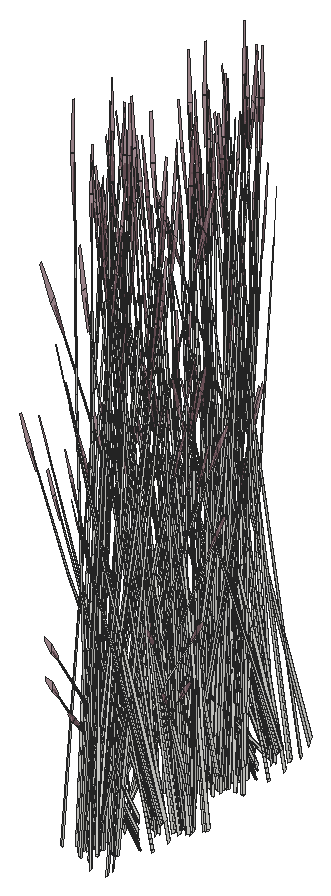
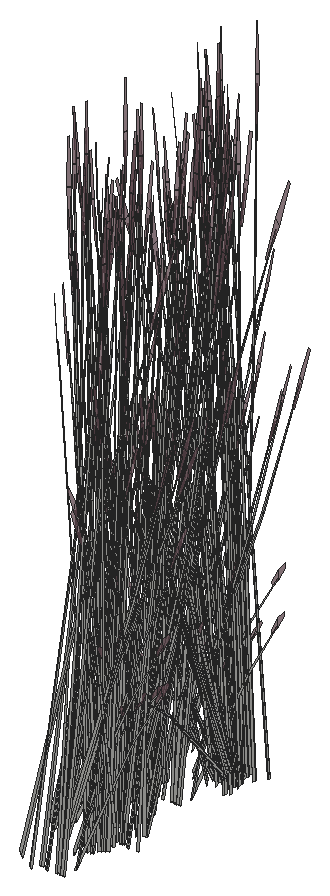
# SketchUp Ruby script. Lengths in inches.
U = 1.inch
M = Sketchup.active_model
def pt(a) = Geom::Point3d.new(a.map { |v| v * U })
def face(e, loops, mat)
  f = e.add_face(loops[0].map { |a| pt(a) })
  loops[1..].each { |l| e.add_face(l.map { |a| pt(a) }).erase! }
  f.material = f.back_material = mat if mat
  f
end
# faces: each face lists its corners as indices into pts; further lists are holes
def faces(e, pts, list, mat = nil) = list.each { |f| face(e, (f[0].is_a?(Array) ? f : [f]).map { |l| l.map { |i| pts[i] } }, mat) }
# xy, xz, yz: faces in a plane at the given z, y or x. An outline is a flat list of corners, or four numbers for a rectangle; further outlines are holes
def ring(l) = l.size == 4 ? [[l[0], l[1]], [l[2], l[1]], [l[2], l[3]], [l[0], l[3]]] : l.each_slice(2).to_a
def flat(e, list, mat, &to3) = list.each { |f| face(e, (f[0].is_a?(Array) ? f : [f]).map { |l| ring(l).map { |u, v| to3.(u, v) } }, mat) }
def xy(e, z, list, mat = nil) = flat(e, list, mat) { |x, y| [x, y, z] }
def xz(e, y, list, mat = nil) = flat(e, list, mat) { |x, z| [x, y, z] }
def yz(e, x, list, mat = nil) = flat(e, list, mat) { |y, z| [x, y, z] }
def lines(e, pts, list) = list.each { |a, b| e.add_line(pt(pts[a]), pt(pts[b])) }
# prism: a flat outline (further loops are holes) pulled along v
def prism(e, loops, v, mat = nil)
  f = face(e, loops, mat); d = Geom::Vector3d.new(v.map { |x| x * U })
  f.pushpull(f.normal.samedirection?(d) ? d.length : -d.length)
end
def box(e, o, s, mat = nil) = prism(e, [[o, [o[0] + s[0], o[1], o[2]], [o[0] + s[0], o[1] + s[1], o[2]], [o[0], o[1] + s[1], o[2]]]], [0, 0, s[2]], mat)
def at(x, y, z, deg = 0) = Geom::Transformation.translation(pt([x, y, z])) * Geom::Transformation.rotation(ORIGIN, Z_AXIS, deg.degrees)
def axes(o, x, y, z) = Geom::Transformation.new([*x, 0, *y, 0, *z, 0, *pt(o).to_a, 1])
def part(name) = M.definitions.add(name)
# library, detail: a bought-in or finely detailed component or shape, given as its bounding box
def library(name, o, s) = part(name).tap { |d| box(d.entities, o, s) }
def detail(e, o, s) = box(e.add_group.entities, o, s)
def put(e, d, t, mat = nil) = e.add_instance(d, t).tap { |i| i.material = mat if mat }
def group(e, t, mat = nil) = e.add_group.tap { |g| g.transformation = t; g.material = mat if mat }.entities
root = M.entities
M.materials.add("LightPink_Translucent").color = [144, 107, 117]
M.materials["LightPink_Translucent"].alpha = 0.75
c1 = part("blade")
p = [[2.15,0.21,22],[0,0.17,0],[0.09,0.45,0],[2.18,0.31,22],[2.29,0.31,22],[0.38,0.45,0],
  [2.48,0.24,33],[2.49,0.24,33],[2.48,0.22,33]]
faces(c1.entities,p,[[0,1,2,3],[4,5,2,3],[6,3,4,7],[8,0,3,6]])
c2 = part("seeds")
p = [[0.3,-0.1,1.38],[-0.01,-0.03,1.59],[-0.01,-0.03,0.03],[0.14,-0.07,-0.07],[0.29,-0.03,3],[0.15,0.01,3.11]]
faces(c2.entities,p,[[0,1,2,3],[1,0,4,5]],"LightPink_Translucent")
c3 = part("blade with seeds")
put(c3.entities,c1,at(0,0,0))
put(c3.entities,c2,axes([2.4,0.25,30.99],[1.5799,-0.05474,1.17369],[-0.12525,1.92788,0.29478],[-0.07173,-0.02425,1.56792]))
put(root,c3,axes([407.93,42.8,-7.59],[-0.36417,-0.37086,0.447],[0.38674,-0.31985,0.36857],[-0.06718,0.174,0.92496]))
put(root,c3,axes([403.99,46.43,-9.95],[0,-0.62892,0],[0.63949,0,0],[0,0,1.6711]))
put(root,c3,axes([404.77,44.98,-9.69],[-0.47863,-0.27177,0.46235],[0.28609,-0.48733,0],[0.10901,0.0619,1.46668]))
put(root,c3,axes([403.6875,46.04,-9.8],[-0.42403,0.49328,0.42607],[-0.50377,-0.43543,0.16719],[0.10223,-0.04923,1.47927]))
put(root,c3,axes([408.2,49.62,-7.64],[-0.50273,-0.13626,-0.47583],[0.17232,-0.46717,-0.36857],[-0.0461,-0.18809,0.91046]))
put(root,c3,axes([402.95,45.22,-9.7],[-0.14774,0.54019,0.16428],[-0.54062,-0.15287,0.32672],[0.09339,-0.00263,1.49371]))
put(root,c3,axes([407.82,41.85,-8.39],[0.09522,-0.18683,1.59586],[0.39947,0.38663,0.12904],[-0.18021,0.24097,0.68222]))
put(root,c3,axes([404.08,45.83,-9.5625],[0.09866,-0.48509,0.13483],[0.48202,0.0842,-0.38503],[0.08772,0.04981,1.18024]))
put(root,c3,axes([407.3,48.17,-7.62],[-0.00954,0.06515,1.65179],[-0.47055,0.23645,-0.15608],[-0.13847,-0.12087,0.29231]))
put(root,c3,axes([403.875,45.95,-9.47],[-0.30722,-0.45622,0.41661],[0.46535,-0.32126,-0.2005],[0.09942,0.05645,1.33761]))
put(root,c3,axes([407.93,42.91,-7.78],[-0.34603,0.28618,-0.32977],[-0.32756,-0.32677,0.42575],[-0.04984,0.16603,0.81462]))
put(root,c3,axes([406.74,42.82,-7.61],[-0.01271,0.10756,1.62908],[0.36076,0.37419,-0.25764],[-0.09444,0.17695,0.13065]))
put(root,c3,axes([407.2,49.32,-7.26],[0.56969,-0.13971,0.50064],[0.09887,0.54803,0.4128],[-0.13398,-0.16152,1.03595]))
put(root,c3,axes([408.15,44.02,-9.42],[-0.01324,-0.32319,1.06958],[0.33072,0.23052,0.78586],[-0.06504,0.15405,0.23558]))
put(root,c3,axes([408.63,49.59,-7.3125],[-0.50045,0.25306,-0.11324],[-0.24593,-0.44915,-0.62851],[-0.06603,-0.18927,0.95501]))
put(root,c3,axes([406.64,48.83,-9.42],[0.26677,0.18918,1.06958],[-0.38851,0.11372,0.78586],[-0.08313,-0.14539,0.23558]))
put(root,c3,axes([404.03,45.98,-9.52],[0.51635,-0.36087,-0.27094],[0.34336,0.5099,-0.46562],[0.1274,0.05178,1.4872]))
put(root,c3,axes([407.29,49.83,-7.36],[-0.43608,-0.26272,-0.66157],[0.30991,-0.46038,0.07984],[-0.158,-0.15687,0.93586]))
put(root,c3,axes([407.14,49.48,-7.78],[-0.07899,-0.43781,-0.32977],[0.45153,-0.11561,0.42575],[-0.12128,-0.12546,0.81462]))
put(root,c3,axes([404.43,46.57,-9.95],[0.57217,0,0],[0,0.56272,0],[0,0,1.66132]))
put(root,c3,axes([404.59,45.25,-9.7],[-0.54955,0.14427,0.16428],[-0.1357,-0.53689,0.32672],[0.04901,0.07823,1.49371]))
put(root,c3,axes([405.2,45.23,-10.11],[0.12013,0.47362,-0.28847],[-0.47712,0.13449,0.28847],[0.09619,0.05462,1.29413]))
put(root,c3,axes([407.33,49.44,-7.6],[0.23243,-0.34529,0.05988],[0.331,0.20103,0.47138],[-0.10701,-0.1107,0.71878]))
put(root,c3,axes([406.43,49.4,-10.61],[-0.04954,0.0716,1.6421],[-0.50062,0.15438,-0.25086],[-0.12094,-0.14044,0.2797]))
put(root,c3,axes([407.26,51.37,-10.05],[-0.21003,-0.55738,-0.65031],[0.60499,-0.20074,-0.17068],[-0.02321,-0.18874,1.43544]))
put(root,c3,axes([404.24,46.29,-9.78],[-0.64638,-0.11452,0.45814],[0.13155,-0.64678,0.17978],[0.09446,0.06245,1.59061]))
put(root,c3,axes([408.16,42.61,-7.03],[-0.01331,0.50278,-0.73435],[-0.56035,-0.03377,0.08862],[-0.05914,0.213,1.03881]))
put(root,c3,axes([406.7,43.93,-7.62],[0.05802,-0.03282,1.65179],[0.47954,0.21828,-0.15608],[-0.01127,0.18175,0.29231]))
put(root,c3,axes([404.35,47.82,-9.97],[0.53691,-0.18442,-0.17877],[0.18866,0.53125,0.00007],[0.05927,-0.02038,1.61933]))
put(root,c3,axes([407.08,49.84,-7.64],[-0.50465,0.12921,-0.47583],[-0.08828,-0.48932,-0.36857],[-0.13555,-0.14022,0.91046]))
put(root,c3,axes([404.41,46.82,-9.9375],[0.35699,0.35109,0],[-0.35699,0.35109,0],[0,0,1.57621]))
put(root,c3,axes([405.38,46.66,-9.7],[-0.40181,-0.39593,0.16428],[0.40492,-0.38402,0.32672],[-0.04438,0.08086,1.49371]))
put(root,c3,axes([407.77,43.73,-9.59],[0.16138,-0.08575,1.33163],[0.39845,0.25854,-0.28638],[-0.1186,0.22371,0.56934]))
put(root,c3,axes([407.88,49.11,-10.02],[-0.35341,0.31182,-0.03625],[-0.32382,-0.34152,-0.16435],[-0.0228,-0.09677,0.54209]))
put(root,c3,axes([404.41,46.4,-9.47],[0.24813,-0.48978,0.41661],[0.51557,0.23571,-0.2005],[0,0.1129,1.33761]))
put(root,c3,axes([404.3125,46.68,-9.87],[0,0.62861,-0.05249],[-0.63949,0,0],[0,0.01975,1.67027]))
put(root,c3,axes([404.36,46.24,-9.94],[0.30722,0.45622,-0.41661],[-0.46535,0.32126,0.2005],[0.09942,0.05645,1.33761]))
put(root,c3,axes([405.71,46.68,-9.69],[0,-0.54355,0.46235],[0.57217,0,0],[0,0.1238,1.46668]))
put(root,c3,axes([408.33,52.8,-8.9],[0.44194,0.21918,1.40854],[-0.43295,0.47219,0.557],[-0.19393,-0.27986,1.18082]))
put(root,c3,axes([404.625,46.52,-9.5625],[0.47648,-0.15851,0.13483],[0.16686,0.45265,-0.38503],[0,0.09962,1.18024]))
put(root,c3,axes([407.4,49.84,-7.3],[0.07899,0.43781,0.32977],[-0.45153,0.11561,-0.42575],[-0.12128,-0.12546,0.81462]))
put(root,c3,axes([406.02,51.29,-10.12],[0,-0.54355,-0.46235],[0.57217,0,0],[0,-0.1238,1.46668]))
put(root,c3,axes([404.19,48.11,-9.95],[0.51557,0.24403,0],[-0.24813,0.50705,0],[0,0,1.62917]))
put(root,c3,axes([406.27,51.3,-10.11],[0.35699,-0.33913,-0.28847],[0.35699,0.33913,0.28847],[0,-0.10923,1.29413]))
put(root,c3,axes([406.12,49.67,-10.02],[-0.14753,0.44383,-0.03625],[-0.45406,-0.13653,-0.16435],[-0.06894,-0.07259,0.54209]))
put(root,c3,axes([407.52,51.92,-9.52],[-0.57594,-0.25935,-0.27094],[0.27732,-0.5474,-0.46562],[-0.0181,-0.1344,1.4872]))
put(root,c3,axes([405.88,51.7,-9.79],[-0.63949,0,0],[0,-0.60749,-0.48057],[0,-0.13836,1.52448]))
put(root,c3,axes([404.01,47.9,-9.87],[0.22235,0.62444,-0.05599],[-0.63531,0.21881,0],[0.00776,0.02181,1.60327]))
put(root,c3,axes([406.1,46.77,-9.79],[0.63949,0,0],[0,0.60749,-0.48057],[0,0.13836,1.52448]))
put(root,c3,axes([405.84,47.08,-9.95],[-0.63917,-0.00435,-0.04634],[0,-0.60749,0.46507],[-0.02009,0.13829,1.47457]))
put(root,c3,axes([404.46,46.55,-9.52],[0.57594,0.25935,-0.27094],[-0.27732,0.5474,-0.46562],[0.0181,0.1344,1.4872]))
put(root,c3,axes([405.71,47.17,-10.11],[-0.35699,0.33913,-0.28847],[-0.35699,-0.33913,0.28847],[0,0.10923,1.29413]))
put(root,c3,axes([404.4,46.96,-9.94],[-0.24813,0.48978,-0.41661],[-0.51557,-0.23571,0.2005],[0,0.1129,1.33761]))
put(root,c3,axes([406.37,51.54,-9.83],[-0.47569,0.45698,0.2864],[-0.47598,-0.45217,-0.33981],[-0.01661,-0.12977,1.53541]))
put(root,c3,axes([407.66,52.49,-9.73],[0.13555,-0.64407,-0.21817],[0.64269,0.11227,0.47743],[-0.1123,-0.08895,1.45677]))
put(root,c3,axes([404.26,48.53,-7.3],[-0.07899,-0.43781,0.32977],[0.45153,-0.11561,-0.42575],[0.12128,0.12546,0.81462]))
put(root,c3,axes([405.96,47.18,-10.12],[0,0.54355,-0.46235],[-0.57217,0,0],[0,0.1238,1.46668]))
put(root,c3,axes([404.5625,46.01,-7.83],[-0.44191,-0.28242,1.28769],[0.46662,-0.43971,0.5556],[0.14258,0.26499,1.24467]))
put(root,c3,axes([406.27,51.79,-9.69],[0,0.54355,0.46235],[-0.57217,0,0],[0,-0.1238,1.46668]))
put(root,c3,axes([407.62,52.23,-9.94],[-0.30722,-0.45622,-0.41661],[0.46535,-0.32126,0.2005],[-0.09942,-0.05645,1.33761]))
put(root,c3,axes([405.23,48.31,-9.42],[-0.28795,-0.15629,1.06958],[0.37181,-0.1588,0.78586],[0.10029,0.13452,0.23558]))
put(root,c3,axes([407.57,52.07,-9.47],[-0.24813,0.48978,0.41661],[-0.51557,-0.23571,-0.2005],[0,-0.1129,1.33761]))
put(root,c3,axes([403.82,49.14,-7.62],[0.00151,-0.06581,1.65179],[0.43826,-0.29033,-0.15608],[0.15223,0.10363,0.29231]))
put(root,c3,axes([404.69,47.11,-10.05],[0.18752,0.49766,-0.6445],[-0.54017,0.17923,-0.16915],[0.02073,0.16852,1.42262]))
put(root,c3,axes([403.18,48.6,-7.3],[0.15418,-0.41799,0.32977],[0.44981,0.12192,-0.42575],[0.04124,0.16829,0.81462]))
put(root,c3,axes([405.28,49.02,-9.52],[-0.32795,-0.01705,0.97832],[0.21658,-0.36206,0.54015],[0.12956,0.12863,0.76741]))
put(root,c3,axes([407.74,52.18,-9.8],[0.64638,0.11452,0.42607],[-0.13155,0.64678,0.16719],[-0.09446,-0.06245,1.47927]))
put(root,c3,axes([404.33,48.93,-7.6],[-0.23243,0.34529,0.05988],[-0.331,-0.20103,0.47138],[0.10701,0.1107,0.71878]))
put(root,c3,axes([403.78,50.09,-6.74],[0.35341,-0.31182,-0.06041],[0.32382,0.34152,-0.27392],[0.0228,0.09677,0.90349]))
put(root,c3,axes([404.43,48.83,-7.59],[-0.50866,0.12474,0.447],[-0.08828,-0.48932,0.36857],[0.11963,0.14421,0.92496]))
put(root,c3,axes([406.78,53.24,-10.11],[-0.12013,-0.47362,-0.28847],[0.47712,-0.13449,0.28847],[-0.09619,-0.05462,1.29413]))
put(root,c3,axes([404.2,48.14,-9.59],[0.00902,-0.18018,1.33163],[0.43127,-0.20126,-0.28638],[0.13313,0.21566,0.56934]))
put(root,c3,axes([406.64,53.45,-10.12],[-0.47863,-0.27177,-0.46235],[0.28609,-0.48733,0],[-0.10901,-0.0619,1.46668]))
put(root,c3,axes([403.03,48.77,-7.3125],[0.50045,-0.25306,-0.11324],[0.24593,0.44915,-0.62851],[0.06603,0.18927,0.95501]))
put(root,c3,axes([407.94,52.49,-9.52],[-0.51635,0.36087,-0.27094],[-0.34336,-0.5099,-0.46562],[-0.1274,-0.05178,1.4872]))
put(root,c3,axes([405.96,56.57,-7.36],[-0.24409,-0.44196,-0.66157],[0.50245,-0.2463,0.07984],[-0.05708,-0.21354,0.93586]))
put(root,c3,axes([405.54,55.59,-10.61],[-0.08578,0.01958,1.6421],[-0.47437,-0.22044,-0.25086],[0.00796,-0.18387,0.2797]))
put(root,c3,axes([407.89,52.64,-9.5625],[-0.09866,0.48509,0.13483],[-0.48202,-0.0842,-0.38503],[-0.08772,-0.04981,1.18024]))
put(root,c3,axes([403.46,48.75,-7.64],[0.50273,0.13626,-0.47583],[-0.17232,0.46717,-0.36857],[0.0461,0.18809,0.91046]))
put(root,c3,axes([403.74,47.79,-8.39],[-0.1169,-0.17452,1.59586],[0.54019,-0.14692,0.12904],[0.12209,0.27397,0.68222]))
put(root,c3,axes([406.01,56.19,-7.78],[0.15418,-0.41799,-0.32977],[0.44981,0.12192,0.42575],[-0.04124,-0.16829,0.81462]))
put(root,c3,axes([407.65,55.83,-7.62],[-0.05194,0.04152,1.65179],[-0.50886,-0.14007,-0.15608],[-0.01842,-0.18118,0.29231]))
put(root,c3,axes([405.78,56.48,-7.64],[-0.50273,-0.13626,-0.47583],[0.17232,-0.46717,-0.36857],[-0.0461,-0.18809,0.91046]))
put(root,c3,axes([406.09,55.3125,-9.42],[0.06561,0.31695,1.06958],[-0.36394,-0.17555,0.78586],[0.03916,-0.16229,0.23558]))
put(root,c3,axes([408.52,52.65,-9.7],[-0.49938,-0.43748,-0.23459],[0.42021,-0.49126,0.51337],[-0.13447,0.05118,1.56642]))
put(root,c3,axes([407.21,53.49,-9.69],[0.47863,0.27177,0.46235],[-0.28609,0.48733,0],[-0.10901,-0.0619,1.46668]))
put(root,c3,axes([403.28,48.66,-7.36],[0.24409,0.44196,-0.66157],[-0.50245,0.2463,0.07984],[0.05708,0.21354,0.93586]))
put(root,c3,axes([406.93,53.77,-9.79],[-0.31974,0.54466,0],[-0.53494,-0.30375,-0.48057],[-0.12184,-0.06918,1.52448]))
put(root,c3,axes([406.07,56.29,-7.59],[0.50393,0.1421,0.447],[-0.17232,0.46717,0.36857],[-0.03028,-0.18372,0.92496]))
put(root,c3,axes([406.21,56.46,-7.3125],[-0.50045,0.25306,-0.11324],[-0.24593,-0.44915,-0.62851],[-0.06603,-0.18927,0.95501]))
put(root,c3,axes([407.25,57.03,-7.3125],[-0.56206,-0.02693,-0.11324],[0.01536,-0.50991,-0.62851],[0.03904,-0.19638,0.95501]))
put(root,c3,axes([406.2,56.26,-7.6],[0.37684,-0.18473,0.05988],[0.18445,0.33686,0.47138],[-0.03639,-0.14849,0.71878]))
put(root,c3,axes([402.91,49.78,-7.61],[0.06483,0.08753,1.62908],[0.52315,0.03439,-0.25764],[0.05261,0.19303,0.13065]))
put(root,c3,axes([408.27,52.56,-9.94],[-0.55535,0.03355,-0.41661],[-0.05022,-0.55698,0.2005],[-0.09942,0.05645,1.33761]))
put(root,c3,axes([408.89,53.85,-9.96],[-0.31576,-0.54657,-0.04789],[0.53494,-0.30375,0.48057],[-0.13182,0.05204,1.52373]))
put(root,c3,axes([404.83,58.23,-10.05],[-0.21003,-0.55738,-0.65031],[0.60499,-0.20074,-0.17068],[-0.02321,-0.18874,1.43544]))
put(root,c3,axes([406.06,56.64,-7.3],[-0.15418,0.41799,0.32977],[-0.44981,-0.12192,-0.42575],[-0.04124,-0.16829,0.81462]))
put(root,c3,axes([408.74,53.78,-10.11],[-0.47712,-0.13449,-0.28847],[0.12013,-0.47362,0.28847],[-0.09619,0.05462,1.29413]))
put(root,c3,axes([404.75,56.63,-9.79],[-0.31974,-0.54466,0],[0.53494,-0.30375,-0.48057],[0.12184,-0.06918,1.52448]))
put(root,c3,axes([406.1,52.45,-7.3],[0.44516,-0.07768,0.32977],[0.11755,0.44407,-0.42575],[-0.12757,0.11927,0.81462]))
put(root,c3,axes([405.45,55.97,-10.02],[-0.35341,0.31182,-0.03625],[-0.32382,-0.34152,-0.16435],[-0.0228,-0.09677,0.54209]))
put(root,c3,axes([408.66,52.41,-9.52],[0.05959,0.62022,-0.27094],[-0.62068,0.0375,-0.46562],[-0.1093,0.08261,1.4872]))
put(root,c3,axes([405.09,53.71,-6.74],[0.45129,0.14509,-0.06041],[-0.13882,0.44656,-0.27392],[-0.07381,0.0678,0.90349]))
put(root,c3,axes([408.29,52.88,-10.08],[-0.34446,0.40855,-0.58063],[-0.42791,-0.37046,-0.15239],[-0.13803,0.10191,1.28164]))
put(root,c3,axes([408.85,54,-10.12],[-0.47863,0.27177,-0.46235],[-0.28609,-0.48733,0],[-0.10901,0.0619,1.46668]))
put(root,c3,axes([405.87,52.41,-7.3125],[0.47307,0.29971,-0.11324],[-0.27254,0.43404,-0.62851],[-0.13365,0.15087,0.95501]))
put(root,c3,axes([405.15,58.375,-9.94],[0.24813,-0.48978,-0.41661],[0.51557,0.23571,0.2005],[0,-0.1129,1.33761]))
put(root,c3,axes([403.84,58.16,-10.11],[0.35699,-0.33913,-0.28847],[0.35699,0.33913,0.28847],[0,-0.10923,1.29413]))
put(root,c3,axes([405.09,58.78,-9.52],[-0.57594,-0.25935,-0.27094],[0.27732,-0.5474,-0.46562],[-0.0181,-0.1344,1.4872]))
put(root,c3,axes([406.7,53.33,-7.3],[0.34603,-0.28618,0.32977],[0.32756,0.32677,-0.42575],[-0.04984,0.16603,0.81462]))
put(root,c3,axes([409.02,51.76,-9.35],[-0.01397,-0.51177,1.31553],[0.63227,0.13266,0.557],[-0.14954,0.28003,1.24175]))
put(root,c3,axes([406.38,53.59,-7.6],[-0.42027,-0.02533,0.05988],[0.01152,-0.38243,0.47138],[-0.04398,0.14649,0.71878]))
put(root,c3,axes([406.52,53.625,-7.59],[-0.36417,-0.37086,0.447],[0.38674,-0.31985,0.36857],[-0.06718,0.174,0.92496]))
put(root,c3,axes([405.46,58.62,-9.73],[0.57623,0.26344,0.22409],[-0.27732,0.5474,0.46562],[0,-0.12618,1.49497]))
put(root,c3,axes([406.52,53.74,-7.78],[-0.34603,0.28618,-0.32977],[-0.32756,-0.32677,0.42575],[-0.04984,0.16603,0.81462]))
put(root,c3,axes([406.48,53.41,-6.97],[0.56206,0.02693,-0.12569],[-0.01536,0.50991,-0.69765],[-0.03904,0.19638,1.06006]))
put(root,c3,axes([405.28,58.25,-9.47],[-0.55535,0.03355,0.41661],[-0.05022,-0.55698,-0.2005],[0.09942,-0.05645,1.33761]))
put(root,c3,axes([406.74,54.85,-9.42],[-0.01324,-0.32319,1.06958],[0.33072,0.23052,0.78586],[-0.06504,0.15405,0.23558]))
put(root,c3,axes([405.26,58.45,-9.8],[0.22235,0.6078,0.42607],[-0.63531,0.21135,0.16719],[0.00776,-0.11168,1.47927]))
put(root,c3,axes([405.14,58.93,-9.47],[-0.24813,0.48978,0.41661],[-0.51557,-0.23571,-0.2005],[0,-0.1129,1.33761]))
put(root,c3,axes([406.86,53.6,-7.34],[0.3661,0.36521,-0.52818],[-0.38674,0.31985,-0.40911],[-0.0557,0.18556,1.01061]))
put(root,c3,axes([406.06,58.5,-9.95],[0,-0.62892,0],[0.63949,0,0],[0,0,1.6711]))
put(root,c3,axes([406.46,54.15,-9.37],[0.46459,-0.09625,0.0606],[0.10681,0.38778,-0.80367],[-0.02945,0.1963,0.72038]))
put(root,c3,axes([406.96,62.42,-8.39],[0.1169,0.17452,1.59586],[-0.54019,0.14692,0.12904],[-0.12209,-0.27397,0.68222]))
put(root,c3,axes([405.75,58.11,-9.8],[-0.42403,0.49328,0.42607],[-0.50377,-0.43543,0.16719],[0.10223,-0.04923,1.47927]))
put(root,c3,axes([407.85,61.26,-7.61],[-0.07822,-0.07621,1.62908],[-0.52201,0.04832,-0.25764],[-0.08331,-0.18228,0.13065]))
put(root,c3,axes([406.22,58.99,-9.86],[-0.47569,-0.46784,-0.05709],[0.47598,-0.46812,0],[-0.01661,-0.01634,1.63492]))
put(root,c3,axes([408.4,62.55,-7.36],[-0.24409,-0.44196,-0.66157],[0.50245,-0.2463,0.07984],[-0.05708,-0.21354,0.93586]))
put(root,c3,axes([405.02,57.29,-9.7],[-0.14774,0.54019,0.16428],[-0.54062,-0.15287,0.32672],[0.09339,-0.00263,1.49371]))
put(root,c3,axes([406.75,53.44,-7.03],[-0.01331,0.50278,-0.73435],[-0.56035,-0.03377,0.08862],[-0.05914,0.213,1.03881]))
put(root,c3,axes([405.28,54.76,-7.62],[0.05802,-0.03282,1.65179],[0.47954,0.21828,-0.15608],[-0.01127,0.18175,0.29231]))
put(root,c3,axes([406.81,61.96,-9.59],[-0.03097,0.17781,1.33163],[-0.45273,0.14885,-0.28638],[-0.10583,-0.22982,0.56934]))
put(root,c3,axes([407.28,53.08,-8.39],[-0.01252,-0.20862,1.59586],[0.54251,0.1384,0.12904],[-0.03356,0.2973,0.68222]))
put(root,c3,axes([405.3125,59.05,-9.8],[0.64638,0.11452,0.42607],[-0.13155,0.64678,0.16719],[-0.09446,-0.06245,1.47927]))
put(root,c3,axes([406.35,54.5625,-9.59],[0.16138,-0.08575,1.33163],[0.39845,0.25854,-0.28638],[-0.1186,0.22371,0.56934]))
put(root,c3,axes([404.96,60.08,-9.7],[0.54955,-0.14427,0.16428],[0.1357,0.53689,0.32672],[-0.04901,-0.07823,1.49371]))
put(root,c3,axes([408.21,62.46,-7.64],[-0.50273,-0.13626,-0.47583],[0.17232,-0.46717,-0.36857],[-0.0461,-0.18809,0.91046]))
put(root,c3,axes([406.65,57.32,-9.7],[-0.54955,0.14427,0.16428],[-0.1357,-0.53689,0.32672],[0.04901,0.07823,1.49371]))
put(root,c3,axes([407.31,61.01,-7.62],[-0.00954,0.06515,1.65179],[-0.47055,0.23645,-0.15608],[-0.13847,-0.12087,0.29231]))
put(root,c3,axes([407.21,62.17,-7.26],[0.56969,-0.13971,0.50064],[0.09887,0.54803,0.4128],[-0.13398,-0.16152,1.03595]))
put(root,c3,axes([406.56,54.14,-8.87],[0.01124,-0.2806,1.43727],[0.50537,0.14821,0.19862],[-0.04379,0.29905,0.67868]))
put(root,c3,axes([406.3,58.36,-9.78],[-0.64638,-0.11452,0.45814],[0.13155,-0.64678,0.17978],[0.09446,0.06245,1.59061]))
put(root,c3,axes([405.79,59.95,-9.95],[-0.16686,-0.46861,0],[0.47648,-0.16411,0],[0,0,1.4375]))
put(root,c3,axes([408.64,62.43,-7.3125],[-0.50045,0.25306,-0.11324],[-0.24593,-0.44915,-0.62851],[-0.06603,-0.18927,0.95501]))
put(root,c3,axes([406.65,61.67,-9.42],[0.26677,0.18918,1.06958],[-0.38851,0.11372,0.78586],[-0.08313,-0.14539,0.23558]))
put(root,c3,axes([407.3,62.67,-7.36],[-0.43608,-0.26272,-0.66157],[0.30991,-0.46038,0.07984],[-0.158,-0.15687,0.93586]))
put(root,c3,axes([407.15,62.32,-7.78],[-0.07899,-0.43781,-0.32977],[0.45153,-0.11561,0.42575],[-0.12128,-0.12546,0.81462]))
put(root,c3,axes([406.6,60.11,-9.7],[0.14774,-0.54019,0.16428],[0.54062,0.15287,0.32672],[-0.09339,0.00263,1.49371]))
put(root,c3,axes([406.48,58.88,-9.9375],[0.35699,0.35109,0],[-0.35699,0.35109,0],[0,0,1.57621]))
put(root,c3,axes([407.44,58.73,-9.7],[-0.40181,-0.39593,0.16428],[0.40492,-0.38402,0.32672],[-0.04438,0.08086,1.49371]))
put(root,c3,axes([405.67,60.17,-9.95],[-0.51557,-0.24403,0],[0.24813,-0.50705,0],[0,0,1.51513]))
put(root,c3,axes([407.34,62.28,-7.6],[0.23243,-0.34529,0.05988],[0.331,0.20103,0.47138],[-0.10701,-0.1107,0.71878]))
put(root,c3,axes([406.44,62.24,-10.61],[-0.04954,0.0716,1.6421],[-0.50062,0.15438,-0.25086],[-0.12094,-0.14044,0.2797]))
put(root,c3,axes([406.47,58.47,-9.47],[0.24813,-0.48978,0.41661],[0.51557,0.23571,-0.2005],[0,0.1129,1.33761]))
put(root,c3,axes([407.27,64.21,-10.05],[-0.21003,-0.55738,-0.65031],[0.60499,-0.20074,-0.17068],[-0.02321,-0.18874,1.43544]))
put(root,c3,axes([406.38,58.75,-9.87],[0,0.62861,-0.05249],[-0.63949,0,0],[0,0.01975,1.67027]))
put(root,c3,axes([407.09,62.68,-7.64],[-0.50465,0.12921,-0.47583],[-0.08828,-0.48932,-0.36857],[-0.13555,-0.14022,0.91046]))
put(root,c3,axes([406.34,59.15,-9.47],[0.55535,-0.03355,0.41661],[0.05022,0.55698,-0.2005],[-0.09942,0.05645,1.33761]))
put(root,c3,axes([407.89,61.95,-10.02],[-0.35341,0.31182,-0.03625],[-0.32382,-0.34152,-0.16435],[-0.0228,-0.09677,0.54209]))
put(root,c3,axes([406.26,60.18,-9.95],[0.51557,0.24403,0],[-0.24813,0.50705,0],[0,0,1.62917]))
put(root,c3,axes([406.35,59.39,-9.5625],[0.37783,0.32657,0.13483],[-0.31516,0.36844,-0.38503],[-0.08772,0.04981,1.18024]))
put(root,c3,axes([408.34,65.64,-8.9],[0.44194,0.21918,1.40854],[-0.43295,0.47219,0.557],[-0.19393,-0.27986,1.18082]))
put(root,c3,axes([407.41,62.68,-7.3],[0.07899,0.43781,0.32977],[-0.45153,0.11561,-0.42575],[-0.12128,-0.12546,0.81462]))
put(root,c3,axes([406.03,64.13,-10.12],[0,-0.54355,-0.46235],[0.57217,0,0],[0,-0.1238,1.46668]))
put(root,c3,axes([406.75,60.4,-9.69],[0.47863,-0.27177,0.46235],[0.28609,0.48733,0],[-0.10901,0.0619,1.46668]))
put(root,c3,axes([406.07,59.97,-9.87],[0.22235,0.62444,-0.05599],[-0.63531,0.21881,0],[0.00776,0.02181,1.60327]))
put(root,c3,axes([406.32,60.65,-10.11],[-0.47712,-0.13449,-0.28847],[0.12013,-0.47362,0.28847],[-0.09619,0.05462,1.29413]))
put(root,c3,axes([407.91,59.15,-9.95],[-0.63917,-0.00435,-0.04634],[0,-0.60749,0.46507],[-0.02009,0.13829,1.47457]))
put(root,c3,axes([407.77,59.24,-10.11],[-0.35699,0.33913,-0.28847],[-0.35699,-0.33913,0.28847],[0,0.10923,1.29413]))
put(root,c3,axes([406.24,59.27,-9.52],[0.05959,0.62022,-0.27094],[-0.62068,0.0375,-0.46562],[-0.1093,0.08261,1.4872]))
put(root,c3,axes([406.46,59.03,-9.94],[-0.24813,0.48978,-0.41661],[-0.51557,-0.23571,0.2005],[0,0.1129,1.33761]))
put(root,c3,axes([406.28,64.14,-10.11],[0.35699,-0.33913,-0.28847],[0.35699,0.33913,0.28847],[0,-0.10923,1.29413]))
put(root,c3,axes([406.13,62.51,-10.02],[-0.14753,0.44383,-0.03625],[-0.45406,-0.13653,-0.16435],[-0.06894,-0.07259,0.54209]))
put(root,c3,axes([407.53,64.76,-9.52],[-0.57594,-0.25935,-0.27094],[0.27732,-0.5474,-0.46562],[-0.0181,-0.1344,1.4872]))
put(root,c3,axes([405.89,64.54,-9.79],[-0.63949,0,0],[0,-0.60749,-0.48057],[0,-0.13836,1.52448]))
put(root,c3,axes([406.48,60.43,-9.83],[0.64025,0.17667,0.2864],[-0.16018,0.63149,-0.33981],[-0.10597,0.07904,1.53541]))
put(root,c3,axes([406.38,64.38,-9.83],[-0.47569,0.45698,0.2864],[-0.47598,-0.45217,-0.33981],[-0.01661,-0.12977,1.53541]))
put(root,c3,axes([407.67,65.33,-9.73],[0.13555,-0.64407,-0.21817],[0.64269,0.11227,0.47743],[-0.1123,-0.08895,1.45677]))
put(root,c3,axes([404.27,60.2,-7.3],[0.34603,-0.28618,0.32977],[0.32756,0.32677,-0.42575],[-0.04984,0.16603,0.81462]))
